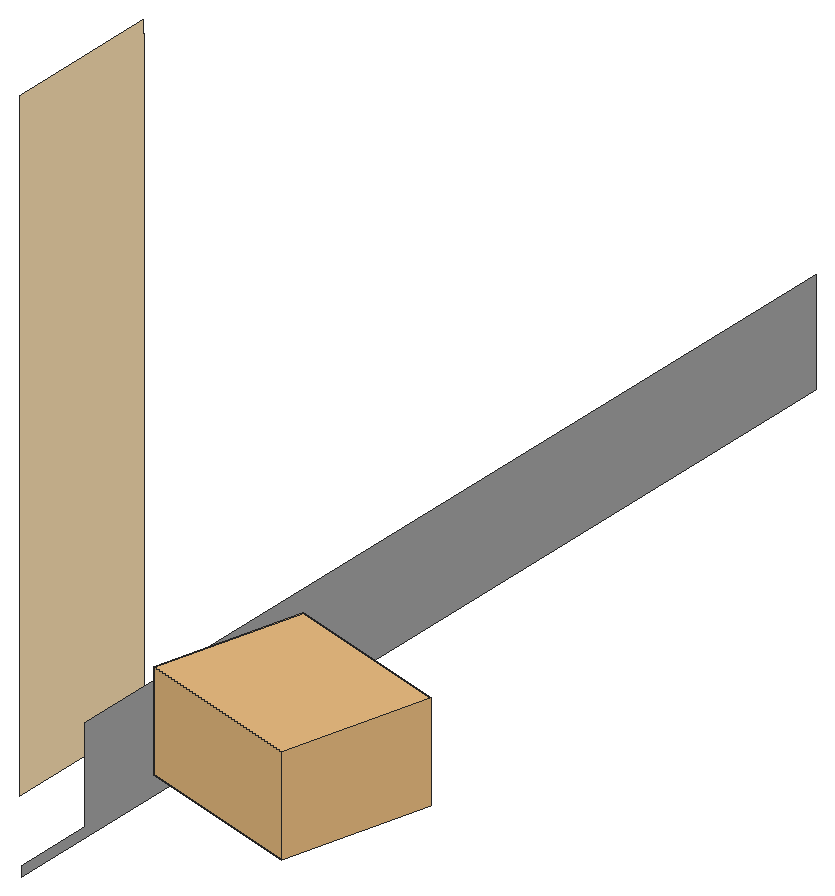
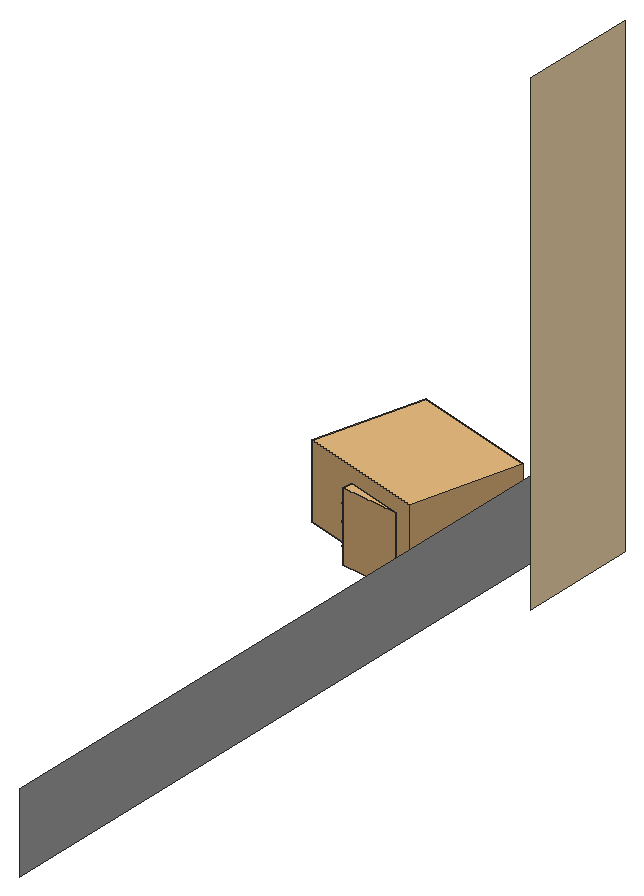
# SketchUp Ruby script. Lengths in inches.
U = 1.inch
M = Sketchup.active_model
def pt(a) = Geom::Point3d.new(a.map { |v| v * U })
def face(e, loops, mat)
  f = e.add_face(loops[0].map { |a| pt(a) })
  loops[1..].each { |l| e.add_face(l.map { |a| pt(a) }).erase! }
  f.material = f.back_material = mat if mat
  f
end
# faces: each face lists its corners as indices into pts; further lists are holes
def faces(e, pts, list, mat = nil) = list.each { |f| face(e, (f[0].is_a?(Array) ? f : [f]).map { |l| l.map { |i| pts[i] } }, mat) }
# xy, xz, yz: faces in a plane at the given z, y or x. An outline is a flat list of corners, or four numbers for a rectangle; further outlines are holes
def ring(l) = l.size == 4 ? [[l[0], l[1]], [l[2], l[1]], [l[2], l[3]], [l[0], l[3]]] : l.each_slice(2).to_a
def flat(e, list, mat, &to3) = list.each { |f| face(e, (f[0].is_a?(Array) ? f : [f]).map { |l| ring(l).map { |u, v| to3.(u, v) } }, mat) }
def xy(e, z, list, mat = nil) = flat(e, list, mat) { |x, y| [x, y, z] }
def xz(e, y, list, mat = nil) = flat(e, list, mat) { |x, z| [x, y, z] }
def yz(e, x, list, mat = nil) = flat(e, list, mat) { |y, z| [x, y, z] }
def lines(e, pts, list) = list.each { |a, b| e.add_line(pt(pts[a]), pt(pts[b])) }
# prism: a flat outline (further loops are holes) pulled along v
def prism(e, loops, v, mat = nil)
  f = face(e, loops, mat); d = Geom::Vector3d.new(v.map { |x| x * U })
  f.pushpull(f.normal.samedirection?(d) ? d.length : -d.length)
end
def box(e, o, s, mat = nil) = prism(e, [[o, [o[0] + s[0], o[1], o[2]], [o[0] + s[0], o[1] + s[1], o[2]], [o[0], o[1] + s[1], o[2]]]], [0, 0, s[2]], mat)
def at(x, y, z, deg = 0) = Geom::Transformation.translation(pt([x, y, z])) * Geom::Transformation.rotation(ORIGIN, Z_AXIS, deg.degrees)
def axes(o, x, y, z) = Geom::Transformation.new([*x, 0, *y, 0, *z, 0, *pt(o).to_a, 1])
def part(name) = M.definitions.add(name)
# library, detail: a bought-in or finely detailed component or shape, given as its bounding box
def library(name, o, s) = part(name).tap { |d| box(d.entities, o, s) }
def detail(e, o, s) = box(e.add_group.entities, o, s)
def put(e, d, t, mat = nil) = e.add_instance(d, t).tap { |i| i.material = mat if mat }
def group(e, t, mat = nil) = e.add_group.tap { |g| g.transformation = t; g.material = mat if mat }.entities
root = M.entities
M.materials.add("0ad16as01f6asdLeafVar1sfd015as60f1as6").color = [231, 235, 211]
M.materials.add("[0032_Moccasin]").color = [255, 228, 181]
M.materials.add("[0132_LightGray]").color = [169, 169, 169]
M.materials.add("asdfasdf0165f6asdLeafVar1sfd015as60f1as6").color = [231, 235, 211]
M.materials.add("dw_stemssadfasdfa0sdf1s01d6w1").color = [90, 97, 50]
c1 = part("vdw_leaf\#2")
p = [[0,0,0],[-2.77,1.61,2.32],[-4.3125,6.1,4.5],[-3.97,13.49,6.09],[-2.47,18.57,6.3],[-0.2,22.73,5.75],
  [2.54,19.66,6.85],[4.3,15.93,7.09],[5.03,7.6,5.43],[3.32,1.76,2.74]]
faces(c1.entities,p,[[0,1,2,3,4,5],[0,5,6,7,8,9]],"asdfasdf0165f6asdLeafVar1sfd015as60f1as6")
c2 = part("dg_branch_1\#2")
p = [[46.12,1.57,35.62],[46,5.42,35.41],[0.14,1.79,0.05],[0.26,-2.0625,0.27],[74.05,2.99,75.8],[74.11,5.28,75.58],
  [103.46,0.47,94.74],[104.03,2.92,94.84],[81.14,16.92,120.46],[81.2,18.78,120.24],[130.47,-5.6875,130.27],[130.58,-3.66,129.85],
  [80.82,34.4375,191.22],[80.64,35.93,190.9],[148.49,-14.56,203.24],[148.9,-12.8125,203.11],[81.08,37.95,226.93],[81.4,39.1,227.03],
  [157.45,-18.19,250.77],[157.7,-17.01,250.41]]
faces(c2.entities,p,[[0,1,2,3],[4,0,1],[4,1,5],[6,4,5],[6,5,7],[8,4,5],[8,5,9],[10,6,7],
  [10,7,11],[12,8,9],[12,9,13],[14,10,11],[14,11,15],[16,12,13],[16,13,17],[18,14,15],
  [18,15,19]],"dw_stemssadfasdfa0sdf1s01d6w1")
c3 = part("vdw_branch1\#3")
put(c3.entities,c1,axes([120.69,-2.42,117.31],[1.12221,-0.24063,-0.65809],[0.19207,1.24776,-0.12871],[0.65778,0.01392,1.11658]))
put(c3.entities,c1,axes([81,38.9,226.05],[0.7888,-0.58155,0],[0.48308,0.65523,0.47],[-0.28484,-0.38635,0.83138]))
put(c3.entities,c1,axes([78.08,12.69,106.05],[-1.43826,-0.02353,-0.03177],[0.0088,-1.31777,0.57755],[-0.03854,0.57714,1.31741]))
put(c3.entities,c1,axes([130.18,-4.73,130.41],[-0.38031,-1.29044,-0.11242],[1.20662,-0.31032,-0.51987],[0.47109,-0.24694,1.24081]))
put(c3.entities,c1,axes([157.08,-17.89,249.93],[-0.91355,0.40674,0],[-0.37496,-0.84216,0.38752],[0.15762,0.35401,0.92186]))
put(c3.entities,c1,axes([90.64,3.03,86.49],[0.32514,-0.85045,-0.99675],[0.69523,0.98247,-0.61148],[1.11061,-0.36604,0.67459]))
put(c3.entities,c1,axes([80.15,28.42,160.95],[-0.16039,0.95636,-1.06292],[-1.41646,0.03966,0.24943],[0.19509,1.07422,0.93709]))
put(c3.entities,c1,axes([126.74,-5.45,129.22],[-0.59819,0.96152,-0.6841],[-0.85772,0.12575,0.92675],[0.75427,0.88089,0.57856]))
put(c3.entities,c1,axes([133.22,-6.12,150.66],[-0.93823,0.76985,0.59124],[-0.47726,-1.08188,0.65135],[0.84525,0.24366,1.02405]))
put(c3.entities,c1,axes([80.43,22.89,141.32],[-1.42571,-0.19312,0.01373],[0.18338,-1.31425,0.5561],[-0.0621,0.5528,1.32692]))
put(c3.entities,c1,axes([33.14,0.88,26.42],[-0.13338,1.31536,0.04876],[-1.04528,-0.13221,0.7073],[0.72315,0.03348,1.07497]))
put(c3.entities,c1,axes([152.63,-15.08,221.76],[-1.28188,0.41945,0.0579],[-0.3638,-1.18547,0.53367],[0.21665,0.49113,1.23869]))
put(c3.entities,c1,axes([80.05,28.28,160.33],[-0.46732,-1.26661,0.40679],[1.27397,-0.40257,0.21004],[-0.07408,0.44645,1.30501]))
put(c3.entities,c1,axes([153.95,-14.8,235.875],[0.39005,1.07743,0.20605],[-0.96443,0.25296,0.50293],[0.42961,-0.3464,0.99807]))
put(c3.entities,c1,axes([80.2,24.22,141.74],[1.33062,-0.46576,0.02628],[0.44746,1.2746,-0.06608],[-0.00197,0.0722,1.37936]))
put(c3.entities,c1,axes([145.48,-12.5,188.92],[-1.32952,0.16983,0.16138],[-0.09299,-1.2361,0.53471],[0.21503,0.51548,1.22904]))
put(c3.entities,c1,axes([139.64,-9.18,171.24],[0.05682,1.30088,0.23414],[-1.13176,-0.05343,0.57151],[0.58357,-0.22963,1.13417]))
put(c3.entities,c1,axes([70.95,4.35,71.98],[-1.1081,-0.41873,0.64752],[0.33675,-1.28259,-0.25313],[0.6937,-0.04625,1.15721]))
put(c3.entities,c1,axes([59.85,4.55,56.17],[-0.26797,1.24526,0.35754],[-0.9369,-0.41634,0.74783],[0.83377,-0.10389,0.98674]))
put(c3.entities,c1,axes([33.11,3.36,25.66],[-0.57817,-1.07968,-0.5679],[1.11554,-0.21356,-0.7297],[0.49375,-0.78178,0.98363]))
put(c3.entities,c2,at(-0.21,0.34,-0.17),"dw_stemssadfasdfa0sdf1s01d6w1")
put(c3.entities,c1,axes([80.91,19.01,122.53],[-0.84258,1.13222,-0.27981],[-1.15093,-0.75138,0.42537],[0.18861,0.47293,1.3457]))
put(c3.entities,c1,axes([119.8,-1.22,114.1],[-1.3235,-0.25012,0.09101],[0.25933,-1.31572,0.15537],[0.05991,0.1698,1.33794]))
put(c3.entities,c1,axes([46.29,5.1,38.04],[0.98937,0.73827,-0.47585],[-0.72359,1.03721,0.10473],[0.44068,0.18581,1.20453]))
put(c3.entities,c1,axes([81.1875,33.03,184.45],[1.33883,0.26986,0.35053],[-0.09581,1.22087,-0.57399],[-0.42216,0.53228,1.20262]))
put(c3.entities,c1,axes([80.16,36.28,206.98],[-0.83993,0.85737,-0.6234],[-1.05964,-0.65701,0.5241],[0.02941,0.81391,1.07976]))
put(c3.entities,c1,axes([154.86,-16.15,234.87],[0.02509,-1.15302,-0.28506],[1.1487,-0.04894,0.29908],[-0.30202,-0.28195,1.11384]))
put(c3.entities,c1,axes([108.77,-0.33,101.14],[-0.47691,-1.03266,-0.72709],[1.25395,-0.29455,-0.40416],[0.15052,-0.81814,1.06325]))
put(c3.entities,c1,axes([89.79,3.01,85.87],[-0.61344,0.75518,0.8965],[-0.17758,-1.01824,0.73622],[1.13385,0.22574,0.58569]))
put(c3.entities,c1,axes([81.56,20.31,123.29],[0.37259,-1.3435,0.21057],[1.29385,0.32364,-0.22445],[0.16906,0.25791,1.34638]))
put(c3.entities,c1,axes([46.45,1.82,36.74],[-0.77883,0.29892,1.0614],[0.19124,-1.24314,0.49044],[1.08598,0.43329,0.67484]))
put(c3.entities,c1,axes([71.37,4.02,72.32],[0.72905,0.81546,-0.74421],[-0.66805,0.98958,0.42988],[0.8391,0.14186,0.97745]))
put(c3.entities,c1,axes([136.59,-5.88,150.53],[0.85845,-0.99897,-0.12437],[0.96526,0.81273,0.13453],[-0.02572,-0.18182,1.28292]))
put(c3.entities,c1,axes([80.375,38.8,225.86],[-0.25178,0.96778,0],[-0.89216,-0.23211,0.38752],[0.37503,0.09757,0.92186]))
put(c3.entities,c1,axes([74.43,7.99,85.38],[-1.05703,0.91669,-0.33543],[-0.95806,-0.87958,0.61531],[0.18697,0.6754,1.25659]))
put(c3.entities,c1,axes([76.57,9.74,89.32],[0.63146,-1.21538,0.33508],[1.18148,0.49387,-0.43517],[0.26321,0.48577,1.26593]))
put(c3.entities,c1,axes([81.6875,36.97,207.4],[0.09422,-1.04424,0.38486],[1.01646,0.1939,0.27727],[-0.33299,0.33382,0.98727]))
put(c3.entities,c1,axes([157.29,-17.17,249.98],[0.50586,-0.50586,0],[0.38853,0.38853,0.41105],[-0.29684,-0.29684,0.56115]))
put(c3.entities,c1,axes([79.92,15.8,106.09],[1.03917,-0.29343,-0.90675],[-0.14587,1.22131,-0.5624],[0.92163,0.5191,0.88824]))
put(c3.entities,c1,axes([61.95,3.88,56.26],[0.41243,-1.28546,0],[1.17466,0.37688,-0.54831],[0.5221,0.16751,1.23363]))
put(c3.entities,c1,axes([151.99,-14.79,208.15],[-0.48571,-1.21723,-0.32393],[1.25386,-0.50033,0],[-0.12005,-0.30087,1.31056]))
put(c3.entities,c1,axes([108.44,0.62,102.22],[0.82183,0.96078,0.38967],[-0.62327,0.08618,1.10203],[0.79141,-0.88661,0.51693]))
put(c3.entities,c1,axes([145.6,-10.56,188.62],[1.03241,-0.02554,-0.82693],[0.3944,1.11584,0.45794],[0.70325,-0.61672,0.89706]))
put(c3.entities,c1,axes([78.59,32.3,183.89],[-1.12675,-0.42036,0.43987],[0.5899,-0.98149,0.57312],[0.14901,0.70693,1.05726]))
put(c3.entities,c1,axes([152.08,-13.42,223.37],[0.79993,-0.44251,-0.69938],[0.68456,0.82615,0.26026],[0.41048,-0.60953,0.85515]))
put(c3.entities,c1,axes([140.71,-8.74,170.55],[0.41903,-1.24177,-0.32393],[1.26224,0.33728,0.33986],[-0.23168,-0.40836,1.26573]))
put(c3.entities,c1,axes([149.25,-12.53,205.78],[1.24456,0.38285,0.23414],[-0.42999,1.04826,0.57151],[-0.02056,-0.62679,1.13417]))
c4 = part("vdw_leaf\#3")
p = [[0,0,0],[-2.77,1.61,2.32],[-4.3125,6.1,4.5],[-3.97,13.49,6.09],[-2.47,18.57,6.3],[-0.2,22.73,5.75],
  [2.54,19.66,6.85],[4.3,15.93,7.09],[5.03,7.6,5.43],[3.32,1.76,2.74]]
faces(c4.entities,p,[[0,1,2,3,4,5],[0,5,6,7,8,9]],"asdfasdf0165f6asdLeafVar1sfd015as60f1as6")
c5 = part("dw_brancj_2\#2")
p = [[9.7,-0.22,29.95],[0.23,-1.96,0.34],[-0.05,1.51,0.11],[9.65,1.51,29.46],[18.64,-8.75,84.43],[18.96,-6.63,84.625],
  [1.53,6.02,63.68],[1.42,8.18,63.25],[-10.58,8.77,161.17],[-10.41,9.98,160.68],[26.34,-9.37,211.72],[26.57,-8.28,211.23]]
faces(c5.entities,p,[[0,1,2],[0,2,3],[4,0,3],[4,3,5],[6,0,3],[6,3,7],[8,6,7],[8,7,9],
  [10,4,5],[10,5,11]],"dw_stemssadfasdfa0sdf1s01d6w1")
c6 = part("vdw_branch2\#3")
put(c6.entities,c4,axes([19.53,-5.9,102.42],[1.12377,-0.50004,0],[0.46097,1.03596,0.47664],[-0.19377,-0.43548,1.13389]))
put(c6.entities,c4,axes([-5.89,6.52,109.44],[-1.07209,0.83679,0],[-0.77141,-0.98832,0.52702],[0.32427,0.41545,1.25373]))
put(c6.entities,c4,axes([-0.44,8.23,75.28],[0.88709,-0.9947,0],[0.92159,0.82189,0.33087],[-0.25219,-0.22491,1.26111]))
put(c6.entities,c4,axes([24.71,-8.97,190.81],[-0.82641,0.91101,0],[-0.83983,-0.76184,0.47664],[0.35303,0.32025,1.13389]))
put(c6.entities,c4,axes([-2.29,8.24,91.35],[1.24603,-0.47303,0],[0.43826,1.15445,0.33087],[-0.11993,-0.31592,1.26111]))
put(c6.entities,c4,axes([12.26,-3.11,37.92],[-0.64625,1.02205,0.22511],[-1.04383,-0.61044,-0.22511],[-0.07533,-0.30931,1.18809]))
put(c6.entities,c4,axes([26.17,-9.17,210.27],[-0.99452,-0.10453,0],[0.09636,-0.91681,0.38752],[-0.04051,0.38539,0.92186]))
put(c6.entities,c4,axes([-6.07,9.4,125.35],[-0.90214,-0.98107,0],[0.90896,-0.83583,0.33087],[-0.24874,0.22873,1.26111]))
put(c6.entities,c4,axes([-4.13,7.29,110.58],[0.44715,-1.078,0.64369],[1.05816,0.63649,0.33087],[-0.58725,0.40856,1.09216]))
put(c6.entities,c4,axes([23.91,-8.22,171.96],[0.62307,0.85009,-0.63406],[-0.71531,0.8798,0.47664],[0.78296,0.12729,0.94004]))
put(c6.entities,c5,at(-0.09,0.18,-0.25),"dw_stemssadfasdfa0sdf1s01d6w1")
put(c6.entities,c4,axes([23.34,-9.65,156.59],[-0.31364,-1.00782,0.58216],[1.10369,-0.17062,0.29925],[-0.17137,0.6239,0.98776]))
put(c6.entities,c4,axes([15.03,-3.37,58.83],[-1.05425,-0.00194,0.58442],[-0.14303,-1.11707,-0.26172],[0.55355,-0.3046,0.99755]))
put(c6.entities,c4,axes([-11.625,9.46,160.37],[0.36812,0.92978,0],[-0.85713,0.33936,0.38752],[0.3603,-0.14265,0.92186]))
put(c6.entities,c4,axes([21.32,-8.53,138.72],[1.21379,0.19904,0],[-0.19904,1.21379,0],[0,0,1.23]))
put(c6.entities,c4,axes([22.54,-9.2,141.43],[-1.02887,0.17955,0.60182],[-0.23387,-1.13057,-0.06253],[0.56696,-0.17376,1.02111]))
put(c6.entities,c4,axes([23.9,-8.82,173.84],[-1.14567,-0.37474,0],[0.35918,-1.0981,0.04438],[-0.01409,0.04308,1.17993]))
put(c6.entities,c4,axes([-7.84,8.92,143.59],[-1.26971,0.40522,0],[-0.37543,-1.17638,0.33087],[0.10274,0.32192,1.26111]))
put(c6.entities,c4,axes([19.77,-8.01,85.98],[-0.32405,-1.14591,0.18674],[1.10278,-0.32969,-0.10948],[0.15845,0.14442,1.16117]))
put(c6.entities,c4,axes([-0.62,5.76,76.34],[-0.08879,1.17576,-0.67771],[-1.34525,-0.16582,-0.11144],[-0.17897,0.66309,1.17383]))
put(c6.entities,c4,axes([20.49,-8.22,121.07],[0.39924,-0.78471,-0.8233],[1.08735,0.33121,0.2116],[0.09035,-0.83005,0.83495]))
put(c6.entities,c4,axes([15.15,-3.72,62.9],[1.16251,0.40128,-0.0211],[-0.39924,1.16074,0.07874],[0.0456,-0.06757,1.2273]))
put(c6.entities,c4,axes([20.72,-8.08,120.26],[-0.03693,1.2277,-0.06551],[-1.22944,-0.03698,0],[-0.00197,0.06548,1.22825]))
put(c6.entities,c4,axes([22.58,-8.36,155.57],[-0.56247,1.09386,0],[-1.00839,-0.51852,0.47664],[0.42389,0.21796,1.13389]))
put(c6.entities,c4,axes([3.97,3.13,57.96],[-1.09459,0.76041,0],[-0.72262,-1.0402,-0.1735],[-0.10109,-0.14552,1.29352]))
put(c6.entities,c4,axes([-10.8,9.06,160.75],[-0.66334,-0.72138,0],[0.66835,-0.61458,0.24329],[-0.1829,0.16818,0.92729]))
put(c6.entities,c4,axes([19.06,-9.3125,103.96],[-1.01345,0.25553,-0.60051],[-0.2265,-1.12952,-0.09839],[-0.59598,0.03076,1.01889]))
put(c6.entities,c4,axes([18.07,-6.2,81.7],[-0.56247,1.09386,0],[-1.00839,-0.51852,0.47664],[0.42389,0.21796,1.13389]))
put(c6.entities,c4,axes([12.95,-0.39,43.31],[0.13044,-1.19832,0],[1.11025,0.12085,0.29925],[-0.30382,-0.03307,1.14057]))
put(c6.entities,c4,axes([2.28,8.28,56.18],[1.32413,-0.31027,0],[0.30923,1.31968,-0.11144],[0.02542,0.1085,1.35543]))
put(c6.entities,c4,axes([-7.55,9.96,143.07],[1.34251,-0.21744,0],[0.20045,1.23761,0.52702],[-0.08426,-0.52024,1.25373]))
put(c6.entities,c4,axes([26.15,-8.25,210.66],[0.94661,-0.25364,0],[0.235,0.87703,0.24329],[-0.06431,-0.24,0.92729]))
put(c6.entities,c4,axes([-6.48,11.37,125.16],[0.64635,1.10315,0.46356],[-1.16569,0.46153,0.52702],[0.27017,-0.6478,1.16488]))
put(c6.entities,c4,axes([25.74,-8.35,191.28],[0.13044,-1.19832,0],[1.11025,0.12085,0.29925],[-0.30382,-0.03307,1.14057]))
put(c6.entities,c4,axes([-5.125,7.47,91.6],[-1.10024,0.63688,0.48318],[-0.78682,-1.00808,-0.46292],[0.14137,-0.65404,1.184]))
c7 = part("vdw_leaf\#1")
p = [[0,0,0],[-2.77,1.61,2.32],[-4.3125,6.1,4.5],[-3.97,13.49,6.09],[-2.47,18.57,6.3],[-0.2,22.73,5.75],
  [2.54,19.66,6.85],[4.3,15.93,7.09],[5.03,7.6,5.43],[3.32,1.76,2.74]]
faces(c7.entities,p,[[0,1,2,3,4,5],[0,5,6,7,8,9]],"0ad16as01f6asdLeafVar1sfd015as60f1as6")
c8 = part("dw_branch_3\#2")
p = [[-10.06,-1.6,62.9],[-0.2,1.54,-0.01],[-10.43,1.54,62.72],[0.18,-1.6,0.17],[-23.75,-21.66,88.91],[-25.7,-20.3,89.55],
  [13.4,11.62,104.56],[13.33,13.52,104.47],[-49.25,-41.87,130.3125],[-50.33,-40.21,130.71],[-4.97,21.13,143.98],[35.61,27.99,178.64],
  [-5.09,23.64,143.96],[35.32,29.14,178.46],[-67.7,-55.38,181.06],[-68.34,-54.45,181.62],[-22.8125,33.9,200.59],[-22.94,35.79,200.41],
  [56.61,36.78,229.75],[56.29,38.09,229.57],[-70.63,-67.46,248.85],[-70.72,-66.33,249.5],[-25.05,43.32,240.75],[-24.98,44.26,240.57]]
faces(c8.entities,p,[[0,1,2],[0,3,1],[4,2,5],[4,0,2],[6,0,2],[6,2,7],[8,4,5],[8,5,9],
  [10,6,7],[11,6,7],[10,7,12],[11,7,13],[14,8,9],[14,9,15],[16,10,12],[16,12,17],
  [18,11,13],[18,13,19],[20,14,15],[20,15,21],[22,16,17],[22,17,23]],"dw_stemssadfasdfa0sdf1s01d6w1")
c9 = part("dw_branch3\#2")
put(c9.entities,c7,axes([-70.33,-63.58,233.32],[-1.00752,0.412,0.78596],[-0.24851,-1.22189,0.32195],[0.83141,0.09817,1.01433]))
put(c9.entities,c7,axes([-66.93,-54.91,182.82],[-0.84976,-0.98359,0.33619],[0.99572,-0.74889,0.32577],[-0.05223,0.46521,1.22907]))
put(c9.entities,c7,axes([-46.12,-39.49,126.35],[1.23843,0.5364,0.23552],[-0.56438,0.94474,0.81599],[0.15707,-0.83465,1.07498]))
put(c9.entities,c7,axes([13.0625,13.13,104.77],[-1.01271,0.69982,-0.26884],[-0.74268,-0.99813,0.19939],[-0.10222,0.31872,1.21473]))
put(c9.entities,c7,axes([-18.87,30.42,186.42],[0.36309,1.06515,-0.56675],[-1.14134,0.49515,0.19939],[0.39128,0.45593,1.10754]))
put(c9.entities,c7,axes([-3.2,4.15,75.77],[-1.04153,0.55414,0.44243],[-0.23365,-1.01045,0.71554],[0.6695,0.50943,0.93801]))
put(c9.entities,c7,axes([23.2,19.41,136.3],[-0.65687,-1.11295,-0.05714],[1.05857,-0.61429,-0.20411],[0.15163,-0.1536,1.24868]))
put(c9.entities,c7,axes([-25.57,35.48,201.32],[-0.64726,0.62827,0.87973],[-0.71635,-1.0172,0.19939],[0.80962,-0.39773,0.87973]))
put(c9.entities,c7,axes([-36.37,-32.14,110.35],[-0.80747,1.09962,0.12544],[-0.83333,-0.50188,-0.96467],[-0.72833,-0.64487,0.96467]))
put(c9.entities,c7,axes([-9.89,26.72,156.79],[0.45529,1.02969,0.56572],[-1.16919,0.33753,0.32662],[0.11537,-0.64297,1.07744]))
put(c9.entities,c7,axes([-26.57,46.1,241.0625],[0.00015,0.80921,0.22536],[-0.83985,0.00446,-0.01542],[-0.01605,-0.22532,0.80906]))
put(c9.entities,c7,axes([-9.2,-2.58,61.06],[-1.10001,-0.40312,0.39014],[0.40883,-1.1116,0.00411],[0.35732,0.13566,1.14763]))
put(c9.entities,c7,axes([-69.91,-63.11,233.93],[1.36249,-0.1432,0],[0.13201,1.25603,0.5309],[-0.05549,-0.52799,1.26295]))
put(c9.entities,c7,axes([32.2,25.46,166.13],[0.06878,-1.29051,-0.05714],[1.22165,0.07415,-0.20411],[0.2113,-0.04403,1.24868]))
put(c9.entities,c7,axes([-5.68,-0.66,44.43],[-0.48448,-1.12287,0.17078],[0.98138,-0.33653,0.57135],[-0.48308,0.36756,1.04626]))
put(c9.entities,c7,axes([43.45,32.81,198.64],[0.5408,1.19584,0.14106],[-0.94242,0.32409,0.86557],[0.74952,-0.45533,0.98656]))
put(c9.entities,c7,axes([12.52,14.14,104.98],[1.02694,0.54888,0.41092],[-0.53566,1.05407,-0.06927],[-0.38969,-0.12321,1.13846]))
put(c9.entities,c7,axes([44.55,32.375,198.73],[-0.65687,-1.11295,-0.05714],[1.05857,-0.61429,-0.20411],[0.15163,-0.1536,1.24868]))
put(c9.entities,c7,axes([-5.67,21.17,141.44],[-1.10726,0.43603,-0.32953],[-0.49537,-1.03435,0.29588],[-0.17521,0.40597,1.12589]))
put(c9.entities,c7,axes([55.69,37.84,229.48],[0.18984,0.96334,0.18958],[-0.71996,0.0053,0.69399],[0.66755,-0.26823,0.69457]))
put(c9.entities,c7,axes([-21.52,36.85,205.2],[0.72606,-0.98817,0.14519],[0.94364,0.7084,0.10251],[-0.16885,0.05176,1.19664]))
put(c9.entities,c7,axes([-68.51,-56.35,196.07],[1.16319,0.72381,0],[-0.66725,1.0723,0.5309],[0.28049,-0.45075,1.26295]))
put(c9.entities,c8,at(0.01,-0.09,-0.02),"dw_stemssadfasdfa0sdf1s01d6w1")
put(c9.entities,c7,axes([-2.49,5.18,75.91],[0.78614,-0.90346,-0.30078],[0.86953,0.79562,-0.11715],[0.28546,-0.14014,1.16705]))
put(c9.entities,c7,axes([-23.125,-16.22,82.25],[0.32175,1.32576,0.12544],[-1.33153,0.31835,0.05068],[0.01989,-0.13382,1.3633]))
put(c9.entities,c7,axes([-23.75,41.99,230.3],[0.85958,-0.87451,0.14519],[0.66531,0.75721,0.62192],[-0.54076,-0.36226,1.01955]))
put(c9.entities,c7,axes([27.07,22.48,149.34],[0.92952,-0.64745,-0.62467],[0.50188,1.074,-0.36637],[0.71693,0.02135,1.04468]))
put(c9.entities,c7,axes([17.66,16.25,119.93],[-0.91649,0.83891,-0.3601],[-0.87434,-0.77966,0.40896],[0.0492,0.54447,1.14321]))
put(c9.entities,c7,axes([-68.37,-54.54,181.63],[0.32047,1.28399,0.35434],[-1.33153,0.31835,0.05068],[-0.03484,-0.35624,1.32241]))
put(c9.entities,c7,axes([-28.98,-27.1,96.48],[-0.8814,-0.35966,-0.98523],[0.75246,-1.11336,-0.26672],[-0.73065,-0.71272,0.91382]))
put(c9.entities,c7,axes([-15.23,28.43,172.72],[-1.21149,0.11898,0.32517],[-0.09739,-1.25259,0.09551],[0.33228,0.0667,1.21356]))
put(c9.entities,c7,axes([-17.5625,31.23,186.85],[-0.49275,-1.12287,0.14519],[0.95014,-0.33653,0.62192],[-0.53717,0.36756,1.01955]))
put(c9.entities,c7,axes([26.7,21.22,149.39],[-1.00104,0.22334,0.83093],[0.36894,-1.0402,0.72406],[0.77731,0.78134,0.72643]))
put(c9.entities,c7,axes([-31.125,-24.87,97.38],[0.75482,-0.86936,0.69068],[-0.00159,0.80023,1.00899],[-1.08766,-0.58016,0.45842]))
put(c9.entities,c7,axes([-71.21,-66.73,248.67],[0.25207,0.96771,0],[-0.8921,0.23237,0.38752],[0.375,-0.09768,0.92186]))
put(c9.entities,c7,axes([-24.11,41.05,229.55],[-1.11612,0.51924,-0.26884],[-0.56394,-1.10897,0.19939],[-0.15444,0.29694,1.21473]))
put(c9.entities,c7,axes([6.75,8.37,91.63],[-0.33418,-1.12287,0.39014],[1.13558,-0.33653,0.00411],[0.10478,0.36756,1.14763]))
put(c9.entities,c7,axes([-26,45.89,241.63],[-0.26986,-0.70824,-0.32129],[0.56818,-0.39091,0.38449],[-0.49365,-0.09775,0.63011]))
put(c9.entities,c7,axes([3.74,17.32,124.35],[0.22441,1.22913,-0.16274],[-1.07812,0.11178,-0.64246],[-0.61228,0.25367,1.07162]))
put(c9.entities,c7,axes([-5.44,22.27,140.88],[1.2203,0.00475,0.31374],[-0.097,1.20386,0.35905],[-0.29841,-0.37189,1.1663]))
put(c9.entities,c7,axes([-13.79,29.35,173.31],[0.83169,-0.90108,0.14519],[0.68877,0.73594,0.62192],[-0.55187,-0.34509,1.01955]))
put(c9.entities,c7,axes([-16.92,-7.26,72.98],[1.30647,0.30378,-0.27886],[0.07026,0.74892,1.14503],[0.40633,-1.10623,0.69861]))
put(c9.entities,c7,axes([4.8,17.55,125.22],[-0.25598,-1.17842,0.26559],[1.01553,-0.08455,0.60363],[-0.56975,0.35087,1.00767]))
put(c9.entities,c7,axes([5.3125,8.35,91.45],[0.00638,1.22913,-0.27714],[-1.16413,0.11178,0.46895],[0.48205,0.25367,1.13617]))
put(c9.entities,c7,axes([38.12,30.57,183.07],[1.12534,0.26182,-0.63833],[-0.46674,1.18829,-0.33545],[0.5081,0.51169,1.10563]))
put(c9.entities,c7,axes([-70.41,-60.38,214.47],[-0.41425,1.30587,0],[-1.20383,-0.38188,0.5309],[0.50605,0.16053,1.26295]))
put(c9.entities,c7,axes([37.03,28.75,180.67],[-1.12533,0.00102,-0.63799],[-0.00113,-1.2408,0],[-0.62497,0.00057,1.10237]))
put(c9.entities,c7,axes([30.71,25.35,165.96],[-0.1364,1.29314,0.22715],[-1.08768,-0.23921,0.70862],[0.73536,-0.11394,1.09026]))
put(c9.entities,c7,axes([-38.05,-30.84,110.67],[-0.31533,-1.27379,-0.2839],[1.018,-0.40311,0.67794],[-0.74394,-0.05723,1.08307]))
put(c9.entities,c7,axes([50.11,34.45,213.36],[-1.05669,0.74401,-0.05714],[-0.616,-0.82138,0.69675],[0.37221,0.60904,1.04705]))
put(c9.entities,c7,axes([-65.32,-58.78,200.07],[-1.14597,-0.19668,-0.6713],[0.21784,-1.26924,0],[-0.64812,-0.11124,1.139]))
put(c9.entities,c7,axes([-53.2,-43.37,143.59],[-0.72817,-1.09167,-0.2839],[0.82127,-0.72411,0.67794],[-0.71934,0.19815,1.08307]))
put(c9.entities,c7,axes([-61.1,-50.25,163.67],[-0.52887,1.19686,-0.30066],[-1.10762,-0.57104,-0.32484],[-0.42634,0.12264,1.23812]))
put(c9.entities,c7,axes([-54.12,-42.96,142.67],[0.32175,1.32576,0.12544],[-1.33153,0.31835,0.05068],[0.01989,-0.13382,1.3633]))
put(c9.entities,c7,axes([22.03,20.08,132.3],[1.17066,0.5058,-0.34078],[-0.35758,1.16671,0.50333],[0.49407,-0.35407,1.17172]))
put(c9.entities,c7,axes([-8.59,26.04,158.21],[-0.49275,-1.12287,0.14519],[0.95014,-0.33653,0.62192],[-0.53717,0.36756,1.01955]))
put(c9.entities,c7,axes([49.92,34.03,213.7],[1.24742,-0.35176,0.25024],[0.42127,1.159,-0.4708],[-0.09426,0.52477,1.20753]))
put(c9.entities,c7,axes([-70.34,-67.02,249.05],[-0.57048,-0.79684,0],[0.73827,-0.52855,0.24329],[-0.20203,0.14464,0.92729]))
put(c9.entities,c7,axes([56.04,36.81,228.63],[0.33451,-0.90845,-0.15237],[0.87636,0.33365,-0.06538],[0.11487,-0.11636,0.94597]))
put(c9.entities,c7,axes([-69.93,-60.58,214.88],[-0.45293,-0.99272,-0.78227],[1.14635,-0.58199,0.07483],[-0.40282,-0.65636,1.06615]))
put(c9.entities,c7,axes([-16.77,-8.59,72.7],[-1.22785,0.11509,0.53076],[-0.24879,-1.22495,-0.30991],[0.46742,-0.38989,1.16587]))
put(c9.entities,c7,axes([18.29,17.18,119.24],[1.19981,-0.45946,0.3029],[0.40159,1.22775,0.27158],[-0.37626,-0.1547,1.25575]))
put(c9.entities,c7,axes([-6.73,-0.68,43.74],[0.05346,1.22913,-0.27201],[-1.22696,0.11178,0.26396],[0.28163,0.25367,1.20164]))
put(c9.entities,c7,axes([-58.57,-48.42,160.98],[0.43385,-1.23789,0.39533],[1.04879,0.57965,0.66404],[-0.76727,0.09236,1.13122]))
put(c9.entities,c7,axes([-23.4,38.49,215.38],[0.06762,1.22913,-0.26884],[-1.23909,0.11178,0.19939],[0.21835,0.25367,1.21473]))
put(c9.entities,c7,axes([-22.21,-16.62,83.17],[-0.72817,-1.09167,-0.2839],[0.82127,-0.72411,0.67794],[-0.71934,0.19815,1.08307]))
put(c9.entities,c7,axes([-45.7,-40.77,126.53],[-1.33715,-0.0713,-0.0976],[0.07167,-1.28508,-0.04314],[-0.09306,-0.0492,1.31098]))
put(c9.entities,c7,axes([-22.39,38.51,216.12],[-0.49275,-1.12287,0.14519],[0.95014,-0.33653,0.62192],[-0.53717,0.36756,1.01955]))
c10 = library("Narrowleaf plant",[-0.44,-0.75,-1.28],[7.48,8.05,9.01])
c11 = library("Broadleaf plant",[0,0,0],[62.33,72.62,41.59])
yz(root,2031.3125,[[228.9375,0,327.5,0,327.5,392.3125,327.3125,392.3125,327.3125,400.3125,228.9375,400.3125]],"[0032_Moccasin]")
yz(root,2076.625,[[173.9375,-6,807.5,-6,807.5,60,224.21,60,224.21,0,173.9375,0]],"[0132_LightGray]")
put(root,c3,axes([2112.47,311.21,2.97],[-0.07583,0.05409,0],[-0.05409,-0.07583,0],[0,0,0.11461]))
put(root,c6,axes([2110.41,310.35,3.23],[-0.06851,-0.04024,-0.04853],[0.04493,-0.07649,0],[-0.03401,-0.01998,0.09777]))
put(root,c6,axes([2110.32,311.26,3.73],[-0.10632,-0.02382,-0.02533],[0.02424,-0.1082,0],[-0.02009,-0.0045,0.13407]))
put(root,c9,axes([2114.42,313.9,5.28],[0.06434,-0.05829,0.02833],[0.05722,0.06809,0.01535],[-0.02555,0.00573,0.10572]))
put(root,c9,axes([2115.23,309.55,0.76],[-0.0835,0.03705,-0.03198],[-0.01833,-0.07755,-0.06358],[-0.04138,-0.04041,0.09269]))
put(root,c9,axes([2113.47,309.13,3.17],[0.11088,0,0],[0,0.11088,0],[0,0,0.13644]))
put(root,c3,axes([2122.76,281.375,2.97],[-0.07583,0.05409,0],[-0.05409,-0.07583,0],[0,0,0.11461]))
put(root,c6,axes([2114.99,312.58,2.375],[0.00659,0.0958,-0.06822],[-0.11062,0.0076,0],[0.0038,0.05531,0.11816]))
put(root,c3,axes([2113.16,309.28,2.97],[0.01294,-0.09448,0],[0.09448,0.01294,0],[0,0,0.11734]))
put(root,c6,axes([2120.61,281.43,3.73],[-0.10632,-0.02382,-0.02533],[0.02424,-0.1082,0],[-0.02009,-0.0045,0.13407]))
put(root,c6,axes([2117.78,309.98,1.88],[0.01852,0.08442,-0.0614],[-0.09748,0.02138,0],[0.01069,0.04874,0.10635]))
put(root,c9,axes([2124.71,284.07,5.28],[0.06434,-0.05829,0.02833],[0.05722,0.06809,0.01535],[-0.02555,0.00573,0.10572]))
put(root,c6,axes([2114.85,309.23,1.76],[0.06689,-0.0646,-0.07431],[0.07703,0.07976,0],[0.04344,-0.04195,0.11443]))
put(root,c6,axes([2118.4,309.53,3.73],[0.10716,0.01972,-0.02533],[-0.02007,0.10905,0],[0.02025,0.00373,0.13407]))
put(root,c3,axes([2116.88,310.48,2.97],[0.07973,0.03352,0],[-0.03352,0.07973,0],[0,0,0.10642]))
put(root,c6,axes([2125.28,282.74,2.375],[0.00659,0.0958,-0.06822],[-0.11062,0.0076,0],[0.0038,0.05531,0.11816]))
put(root,c6,axes([2128.07,280.15,1.88],[0.01852,0.08442,-0.0614],[-0.09748,0.02138,0],[0.01069,0.04874,0.10635]))
put(root,c6,axes([2128.6875,279.69,3.73],[0.10716,0.01972,-0.02533],[-0.02007,0.10905,0],[0.02025,0.00373,0.13407]))
put(root,c3,axes([2127.17,280.65,2.97],[0.07973,0.03352,0],[-0.03352,0.07973,0],[0,0,0.10642]))
put(root,c10,axes([2115.98,314.375,7.7],[6.41217,-0.58355,0],[0.58355,6.41217,0],[0,0,6.43866]))
put(root,c11,axes([2183.37,247.99,8.57],[0.38318,1.43005,0],[-1.43005,0.38318,0],[0,0,1.4805]))
put(root,c3,axes([2173.27,348.5,7.1875],[-0.11019,-0.08184,0],[0.08184,-0.11019,0],[0,0,0.16889]))
put(root,c6,axes([2171.37,274.45,6.3],[0.0097,0.14118,-0.10053],[-0.16302,0.01121,0],[0.0056,0.08151,0.17413]))
put(root,c6,axes([2172.22,345.5,8.3],[-0.01475,-0.15988,-0.03733],[0.16271,-0.01501,0],[-0.00279,-0.03021,0.19757]))
